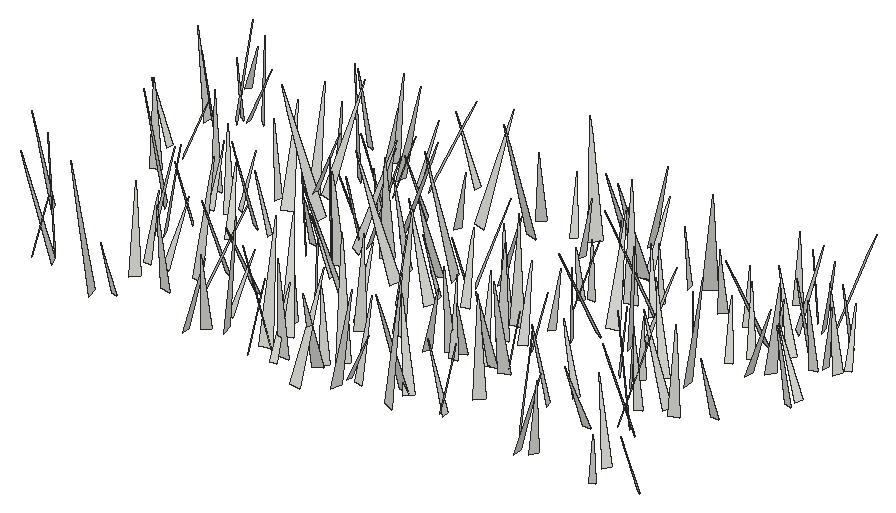
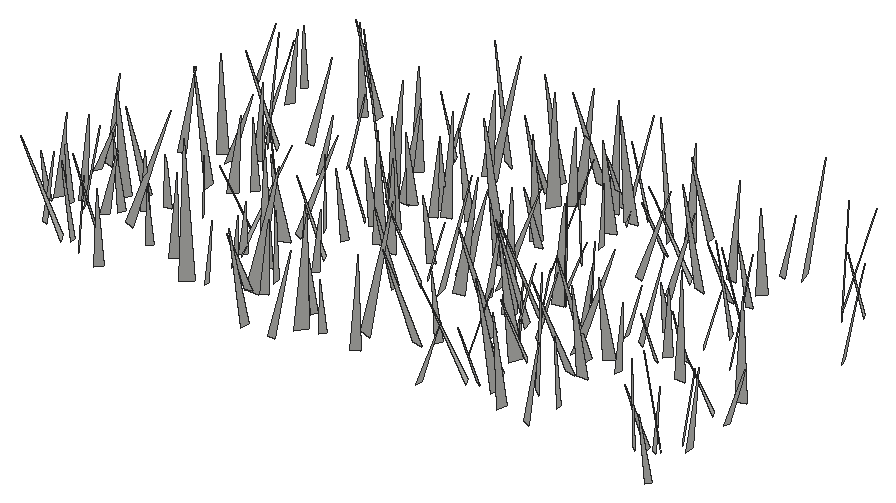
# SketchUp Ruby script. Lengths in inches.
U = 1.inch
M = Sketchup.active_model
def pt(a) = Geom::Point3d.new(a.map { |v| v * U })
def face(e, loops, mat)
  f = e.add_face(loops[0].map { |a| pt(a) })
  loops[1..].each { |l| e.add_face(l.map { |a| pt(a) }).erase! }
  f.material = f.back_material = mat if mat
  f
end
# faces: each face lists its corners as indices into pts; further lists are holes
def faces(e, pts, list, mat = nil) = list.each { |f| face(e, (f[0].is_a?(Array) ? f : [f]).map { |l| l.map { |i| pts[i] } }, mat) }
# xy, xz, yz: faces in a plane at the given z, y or x. An outline is a flat list of corners, or four numbers for a rectangle; further outlines are holes
def ring(l) = l.size == 4 ? [[l[0], l[1]], [l[2], l[1]], [l[2], l[3]], [l[0], l[3]]] : l.each_slice(2).to_a
def flat(e, list, mat, &to3) = list.each { |f| face(e, (f[0].is_a?(Array) ? f : [f]).map { |l| ring(l).map { |u, v| to3.(u, v) } }, mat) }
def xy(e, z, list, mat = nil) = flat(e, list, mat) { |x, y| [x, y, z] }
def xz(e, y, list, mat = nil) = flat(e, list, mat) { |x, z| [x, y, z] }
def yz(e, x, list, mat = nil) = flat(e, list, mat) { |y, z| [x, y, z] }
def lines(e, pts, list) = list.each { |a, b| e.add_line(pt(pts[a]), pt(pts[b])) }
# prism: a flat outline (further loops are holes) pulled along v
def prism(e, loops, v, mat = nil)
  f = face(e, loops, mat); d = Geom::Vector3d.new(v.map { |x| x * U })
  f.pushpull(f.normal.samedirection?(d) ? d.length : -d.length)
end
def box(e, o, s, mat = nil) = prism(e, [[o, [o[0] + s[0], o[1], o[2]], [o[0] + s[0], o[1] + s[1], o[2]], [o[0], o[1] + s[1], o[2]]]], [0, 0, s[2]], mat)
def at(x, y, z, deg = 0) = Geom::Transformation.translation(pt([x, y, z])) * Geom::Transformation.rotation(ORIGIN, Z_AXIS, deg.degrees)
def axes(o, x, y, z) = Geom::Transformation.new([*x, 0, *y, 0, *z, 0, *pt(o).to_a, 1])
def part(name) = M.definitions.add(name)
# library, detail: a bought-in or finely detailed component or shape, given as its bounding box
def library(name, o, s) = part(name).tap { |d| box(d.entities, o, s) }
def detail(e, o, s) = box(e.add_group.entities, o, s)
def put(e, d, t, mat = nil) = e.add_instance(d, t).tap { |i| i.material = mat if mat }
def group(e, t, mat = nil) = e.add_group.tap { |g| g.transformation = t; g.material = mat if mat }.entities
root = M.entities
c1 = part("fur_instance\#9")
p = [[0.8125,0,1.79],[0.67,-0.02,1.48],[0,-0.11,0],[0,0.11,0]]
faces(c1.entities,p,[[0,1,2,3]])
put(root,c1,axes([471.78,258.29,-21.66],[-7.67624,-2.38765,2.18106],[-2.53698,7.93,-0.24775],[2.0054,0.89261,8.03519]))
put(root,c1,axes([502.64,255.98,-21.66],[0.72086,7.11073,0.81641],[7.15729,-0.71063,-0.13028],[0.04812,-0.82534,7.14599]))
put(root,c1,axes([485.32,258.2,-21.66],[5.08569,0.11573,0.95874],[0.07501,-5.17107,0.22632],[-0.96278,0.20845,5.08197]))
put(root,c1,axes([502,260.93,-21.66],[2.77965,-6.05851,0.20454],[-6.05263,-2.78627,-0.276],[-0.3362,0.0706,6.66001]))
put(root,c1,axes([486.8125,259.98,-21.66],[3.24454,-4.71501,1.03025],[-4.7617,-3.32972,-0.24278],[-0.78672,0.70811,5.71834]))
put(root,c1,axes([506.35,258.77,-21.66],[6.38697,-1.69717,1.73981],[-1.81592,-6.58358,0.24416],[-1.61547,0.69051,6.6041]))
put(root,c1,axes([473.87,259.71,-21.66],[-0.63245,-3.70623,0.66325],[-3.76509,0.62047,-0.12308],[-0.01169,0.67448,3.75779]))
put(root,c1,axes([542.48,259.39,-21.66],[1.6475,-3.20979,0.84583],[-3.31321,-1.64761,0.20101],[-0.20196,0.8456,3.6023]))
put(root,c1,axes([493.76,258.83,-21.66],[4.05853,2.67005,1.15678],[2.78357,-4.14094,-0.20805],[-0.84796,-0.81387,4.85361]))
put(root,c1,axes([497.67,260.2,-21.66],[0.14601,-6.62439,2.10053],[-6.94709,-0.08453,0.21629],[0.18059,2.1039,6.62247]))
put(root,c1,axes([531.47,259.7,-21.66],[5.98361,0.11352,0.76596],[0.13466,-6.02993,-0.15823],[-0.76252,-0.17402,5.9826]))
put(root,c1,axes([513.71,258.82,-21.66],[3.41828,7.22194,2.57308],[7.56489,-3.63472,0.1519],[-1.24484,-2.25703,7.98861]))
put(root,c1,axes([533.1875,260.57,-21.66],[4.53528,-3.04969,1.17101],[-3.07507,-4.66168,-0.23091],[-1.10265,0.45689,5.46041]))
put(root,c1,axes([495.05,261.21,-21.66],[-4.80805,-4.95386,1.3489],[-5.02147,4.92244,0.17909],[1.0701,0.84054,6.90116]))
put(root,c1,axes([497.5,258.59,-21.66],[-0.4926,4.67354,0.05511],[4.67276,0.49124,0.10792],[-0.10156,-0.0661,4.69819]))
put(root,c1,axes([513.0625,262.56,-21.66],[-2.01035,-7.12989,1.00319],[-7.18316,2.0575,0.22838],[0.49393,0.90254,7.40437]))
put(root,c1,axes([547.67,261.16,-21.66],[-2.17535,-3.01047,0.60266],[-3.06621,2.16789,-0.23847],[0.15643,0.62897,3.70651]))
put(root,c1,axes([463.9,261.31,-21.66],[-6.35383,-3.10693,1.06991],[-3.1587,6.41685,-0.12448],[0.9057,0.58302,7.07168]))
put(root,c1,axes([488.82,261.16,-21.66],[7.15031,1.42356,2.57616],[1.59453,-7.56218,-0.24693],[-2.47399,-0.75958,7.28646]))
put(root,c1,axes([506.3,261.12,-21.66],[3.59656,-0.31618,0.04156],[-0.31764,-3.59357,0.14939],[-0.02828,0.15246,3.60734]))
put(root,c1,axes([519.87,261.36,-21.66],[-4.57594,-0.69447,0.70937],[-0.73517,4.61906,-0.2203],[0.6671,0.32667,4.62309]))
put(root,c1,axes([461.07,261.14,-21.66],[3.50621,1.98379,0.78234],[2.0421,-3.55715,-0.13217],[-0.61424,-0.50223,4.02634]))
put(root,c1,axes([502.26,261.875,-21.66],[2.60909,-3.89298,2.22887],[-4.24925,-2.97119,-0.21539],[-1.4377,1.71676,4.68148]))
put(root,c1,axes([507.89,260.87,-21.66],[0.83118,5.18677,1.07004],[5.28228,-0.88982,0.21009],[-0.38088,-1.02179,5.24874]))
put(root,c1,axes([519,261.65,-21.66],[-3.23487,-1.73884,2.61208],[-2.22596,3.91581,-0.14997],[2.2117,1.39779,3.66954]))
put(root,c1,axes([494.65,260.86,-21.66],[-1.18605,7.62635,1.82441],[7.84154,1.15487,0.27022],[0.00582,-1.84431,7.7133]))
put(root,c1,axes([513.9,262.27,-21.66],[-4.47005,3.93119,1.60818],[4.11701,4.5843,0.23722],[1.04438,-1.24571,5.94805]))
put(root,c1,axes([462.84,262.94,-21.66],[-5.77727,-4.35757,2.82703],[-4.73437,6.15702,-0.18467],[2.13687,1.8601,7.23403]))
put(root,c1,axes([477.77,263.97,-21.66],[-0.39451,-5.89979,1.57703],[-6.09619,0.47415,0.24879],[0.36204,1.55494,5.90773]))
put(root,c1,axes([528.8,263.52,-21.66],[5.52113,3.74347,2.2115],[4.00437,-5.77059,-0.2291],[-1.6939,-1.44011,6.66663]))
put(root,c1,axes([541.49,263.27,-21.66],[-4.9618,2.41645,1.1014],[2.44275,5.06865,-0.11597],[1.04177,-0.37582,5.51772]))
put(root,c1,axes([503.73,263.29,-21.66],[5.91163,-3.56463,4.13587],[-4.286,-6.80601,0.26026],[-3.38262,2.39395,6.89828]))
put(root,c1,axes([473.07,264.4375,-21.66],[3.99343,-3.31881,2.86458],[-3.84361,-4.5142,0.12826],[-2.10878,1.94301,5.19091]))
put(root,c1,axes([487.09,264,-21.66],[1.39427,3.92432,0.17719],[3.92808,-1.39069,-0.10895],[0.04345,-0.20342,4.16322]))
put(root,c1,axes([495.04,264.1,-21.66],[-2.95766,6.66869,1.17233],[6.76114,2.97762,0.11972],[0.36439,-1.12067,7.29416]))
put(root,c1,axes([520.61,266.57,-21.66],[4.6761,-4.10232,2.76945],[-4.45315,-5.14998,-0.1096],[-2.16064,1.73593,6.21956]))
put(root,c1,axes([533.99,269.05,-21.66],[0.26999,-5.16111,0.17986],[-5.16087,-0.27616,-0.17741],[-0.18667,0.17024,5.16512]))
put(root,c1,axes([493.77,267.14,-21.66],[-4.03311,-0.04964,1.55556],[-0.10181,4.31995,-0.1261],[1.55302,0.15428,4.03144]))
put(root,c1,axes([486.14,270.02,-21.66],[-1.09873,-5.30096,0.04279],[-5.29764,1.09638,-0.20521],[-0.19227,0.08352,5.40974]))
put(root,c1,axes([481.14,266.94,-21.66],[5.4364,3.24485,0.19999],[3.25087,-5.4295,-0.27539],[-0.03035,-0.33899,6.32516]))
put(root,c1,axes([472.36,267.56,-21.66],[0.52075,4.40411,1.27547],[4.58416,-0.47433,-0.2338],[0.09203,-1.29345,4.42863]))
put(root,c1,axes([474.73,267.89,-21.66],[0.96438,4.41888,0.40988],[4.43511,-0.94495,-0.24768],[0.15571,-0.45288,4.5161]))
put(root,c1,axes([479.1,267.98,-21.66],[1.99412,7.08431,1.8343],[7.27705,-2.12036,0.27805],[-0.77249,-1.68678,7.35436]))
put(root,c1,axes([538.9,271.21,-21.66],[-4.24041,-4.62675,0.86788],[-4.65391,4.29598,0.16351],[0.70788,0.52807,6.27385]))
put(root,c1,axes([480.99,271.25,-21.66],[-2.16973,-4.86696,0.63571],[-4.9077,2.16207,-0.19771],[0.07681,0.6613,5.32503]))
put(root,c1,axes([456.41,270.67,-21.66],[-5.55068,-3.03255,1.58004],[-3.06213,5.7489,0.27653],[1.52193,0.50669,6.31901]))
put(root,c1,axes([500.48,270.44,-21.66],[3.75494,-4.9741,2.2471],[-5.32599,-3.93562,0.18806],[-1.1937,1.91308,6.22943]))
put(root,c1,axes([527.41,270.4,-21.66],[-4.67685,-1.64881,1.07356],[-1.71505,4.77313,-0.14071],[0.96421,0.49258,4.95698]))
put(root,c1,axes([509.15,271.6,-21.66],[4.77577,-2.2799,0.31782],[-2.26651,-4.78515,-0.26858],[-0.40236,-0.10607,5.28524]))
put(root,c1,axes([519.17,272.82,-21.66],[2.40943,-6.40182,1.38295],[-6.51779,-2.4885,-0.16399],[-0.64358,1.23501,6.83826]))
put(root,c1,axes([493.33,271.34,-21.66],[2.79577,3.11606,1.7882],[3.42019,-3.00212,-0.11591],[-1.09992,-1.41467,4.18482]))
put(root,c1,axes([517.26,273.11,-21.66],[0.8568,-5.86099,0.80486],[-5.91149,-0.87995,-0.11477],[-0.231,0.77949,5.92218]))
put(root,c1,axes([511.58,272.625,-21.66],[1.49133,-6.04191,1.54576],[-6.23212,-1.50337,0.13646],[-0.23383,1.53405,6.22175]))
put(root,c1,axes([512.8125,273.37,-21.66],[2.32528,-3.90872,0.2043],[-3.90658,-2.33236,-0.15975],[-0.24182,0.09371,4.54527]))
put(root,c1,axes([537.51,272.17,-21.66],[-5.07554,-4.81191,2.50581],[-5.17107,5.32884,-0.24106],[1.64121,1.90882,6.98981]))
put(root,c1,axes([512.68,271.76,-21.66],[-0.37436,4.96388,1.61425],[5.21969,0.34743,0.14211],[-0.02763,-1.62026,4.97594]))
put(root,c1,axes([536.22,271.91,-21.66],[5.52496,2.9641,0.73245],[3.00682,-5.54515,-0.24054],[-0.53047,-0.55942,6.26523]))
put(root,c1,axes([499.2,271.52,-21.66],[-0.62067,4.74172,0.56344],[4.77083,0.63973,-0.12835],[0.20124,-0.5417,4.78044]))
put(root,c1,axes([504.53,272.24,-21.66],[0.76042,7.54721,2.45249],[7.93568,-0.724,-0.23253],[-0.00259,-2.46349,7.58186]))
put(root,c1,axes([495.14,274.3,-21.66],[-6.81995,-3.62088,0.84533],[-3.65528,6.85252,-0.13797],[0.68141,0.51893,7.72033]))
put(root,c1,axes([468.87,272.86,-21.66],[3.65147,4.43575,1.22236],[4.5601,-3.69672,-0.20725],[-0.61278,-1.07778,5.74161]))
put(root,c1,axes([516.36,272.67,-21.66],[-2.91757,4.706,0.99504],[4.75363,2.9987,-0.24403],[0.73452,-0.71423,5.53165]))
put(root,c1,axes([518.86,273.82,-21.66],[3.30079,2.00098,0.99665],[2.11543,-3.37049,-0.23912],[-0.72261,-0.72685,3.85253]))
put(root,c1,axes([528.85,273.5,-21.66],[-4.50468,1.1443,0.55643],[1.12699,4.53841,-0.20945],[0.5907,0.0676,4.64302]))
put(root,c1,axes([469.8,274,-21.66],[5.42096,2.25752,1.64956],[2.38588,-5.61122,-0.16143],[-1.45775,-0.7887,5.87002]))
put(root,c1,axes([536.05,275.6,-21.66],[-1.45922,4.42701,2.15741],[4.90506,1.50733,0.22462],[0.43952,-2.12407,4.65589]))
put(root,c1,axes([540.0625,276.96,-21.66],[2.8988,-5.16102,2.16058],[-5.5292,-3.01461,0.21733],[-0.85564,1.9958,5.91539]))
put(root,c1,axes([470.66,277.77,-21.66],[-3.26871,-2.2439,0.63682],[-2.29753,3.28654,-0.21245],[0.40248,0.53729,3.95909]))
put(root,c1,axes([490.34,277.99,-21.66],[-3.97846,-0.22397,0.26493],[-0.21326,3.98441,0.16592],[0.27363,-0.15114,3.9813]))
put(root,c1,axes([543.85,279.51,-21.66],[0.47232,-5.02453,0.37853],[-5.03579,-0.45765,0.20889],[0.17316,0.39615,5.04235]))
put(root,c1,axes([514.4,278.42,-21.66],[4.01557,-5.25956,2.05629],[-5.53772,-4.16187,0.169],[-1.10676,1.74125,6.61508]))
put(root,c1,axes([500.37,277.47,-21.66],[0.04059,4.23783,1.33242],[4.44047,0.00019,-0.13586],[0.12965,-1.33303,4.23585]))
put(root,c1,axes([538.44,277.81,-21.66],[-5.80532,1.01557,0.17125],[1.00882,5.80466,-0.22508],[0.20737,0.19232,5.88918]))
put(root,c1,axes([465.71,279.17,-21.66],[-6.16765,-3.82155,1.90605],[-3.98751,6.35208,-0.16723],[1.52874,1.15063,7.2537]))
put(root,c1,axes([532.24,278.93,-21.66],[-2.65775,-2.55388,1.91088],[-2.80676,3.05414,0.17806],[1.51521,1.17784,3.68161]))
put(root,c1,axes([476.0625,277.5625,-21.66],[-2.52047,3.62206,0.22803],[3.61381,2.53037,-0.24846],[0.33426,-0.04477,4.40572]))
put(root,c1,axes([489.03,279.4,-21.66],[4.97701,4.02381,2.97396],[4.34378,-5.5566,0.24873],[-2.48337,-1.65505,6.3953]))
put(root,c1,axes([518.21,278.93,-21.66],[2.97809,2.23148,0.68885],[2.24903,-3.04112,0.12836],[-0.62921,-0.30835,3.71915]))
put(root,c1,axes([489.35,280.5,-21.66],[1.40139,-5.88916,2.09043],[-6.21682,-1.53152,-0.14692],[-0.635,1.99706,6.05182]))
put(root,c1,axes([516.77,279.16,-21.66],[-2.07994,4.49979,1.08625],[4.57933,2.1742,-0.23818],[0.67657,-0.88257,4.95151]))
put(root,c1,axes([484.82,280.3,-21.66],[-3.86454,-2.68359,1.87384],[-2.96857,4.09497,-0.25773],[1.3786,1.29506,4.69786]))
put(root,c1,axes([502.83,279.78,-21.66],[-5.78073,2.46703,0.60773],[2.49572,5.79658,0.20851],[0.47643,-0.43109,6.28168]))
put(root,c1,axes([476.64,281.57,-21.66],[-2.84226,-5.05917,1.08036],[-5.16298,2.85167,-0.22901],[0.32566,1.05526,5.79838]))
put(root,c1,axes([529.49,280.45,-21.66],[3.10895,3.01642,1.49943],[3.22004,-3.26039,-0.11754],[-0.98914,-1.13301,4.33019]))
put(root,c1,axes([531.97,281.25,-21.66],[2.86459,-3.18276,1.27512],[-3.34476,-2.95943,0.1272],[-0.754,1.03614,4.28015]))
put(root,c1,axes([479.02,281.16,-21.66],[-3.86057,-0.50737,0.50019],[-0.53854,3.88252,-0.21837],[0.46646,0.28336,3.88764]))
put(root,c1,axes([496.76,281.26,-21.66],[-8.06825,0.70999,0.37952],[0.71569,8.07597,0.10667],[0.36866,-0.13964,8.09873]))
put(root,c1,axes([484.07,282.51,-21.66],[-0.05824,-3.81958,0.55077],[-3.85535,0.08183,0.15984],[0.16986,0.54776,3.81668]))
put(root,c1,axes([502.81,281.625,-21.66],[-3.79015,-1.11399,0.60809],[-1.15598,3.82064,-0.20588],[0.52388,0.37109,3.9451]))
put(root,c1,axes([513.49,282.1,-21.66],[-2.45983,6.23998,3.07468],[6.83629,2.77173,-0.15592],[1.28687,-2.79677,6.7055]))
put(root,c1,axes([506.4,281.81,-21.66],[-1.7521,4.37342,1.24469],[4.49457,1.86786,-0.23622],[0.6891,-1.06311,4.7054]))
put(root,c1,axes([511.42,282.86,-21.66],[-0.9402,5.50023,2.63792],[6.09336,0.97222,0.14463],[0.28664,-2.62629,5.57814]))
put(root,c1,axes([470.32,281.48,-21.66],[0.12612,4.07155,0.3622],[4.08216,-0.1442,0.19951],[-0.2114,-0.35539,4.06861]))
put(root,c1,axes([499.63,285.38,-21.66],[2.0561,-6.44135,0.2848],[-6.4395,-2.06652,-0.24899],[-0.32395,0.19535,6.75697]))
put(root,c1,axes([472.42,282.07,-21.66],[-4.08375,3.22336,1.0157],[3.24667,4.18417,-0.22495],[0.93853,-0.4488,5.19774]))
put(root,c1,axes([520.35,283.38,-21.66],[4.15283,1.56186,1.94961],[1.7605,-4.5132,-0.13443],[-1.7723,-0.82343,4.43479]))
put(root,c1,axes([536.68,283.61,-21.66],[7.17764,0.6661,2.04171],[0.73913,-7.45363,-0.1667],[-2.01642,-0.36113,7.20655]))
put(root,c1,axes([517.06,283.875,-21.66],[3.70956,-2.15387,1.10856],[-2.28011,-3.78925,0.26761],[-0.81802,0.79458,4.28116]))
put(root,c1,axes([496.37,284.1,-21.66],[-5.73495,-0.11109,1.68244],[-0.04447,5.97258,0.24275],[1.68552,-0.22038,5.73089]))
put(root,c1,axes([533.68,283.11,-21.66],[-4.18107,4.06515,1.12452],[4.17237,4.21812,0.26475],[0.61747,-0.97641,5.82552]))
put(root,c1,axes([521.83,286.21,-21.66],[-3.10911,-5.59083,0.18925],[-5.58666,3.11434,0.22319],[0.28707,0.05678,6.39328]))
put(root,c1,axes([492.43,285.25,-21.66],[4.53182,-5.76132,1.66498],[-5.89155,-4.66684,-0.11276],[-1.12014,1.237,7.32923]))
put(root,c1,axes([504.39,284.9,-21.66],[-3.02688,-2.08558,0.64094],[-2.07151,3.09116,0.27563],[0.68504,0.13224,3.66547]))
put(root,c1,axes([459.58,284.98,-21.66],[2.04038,-5.82637,1.87095],[-6.1057,-2.07021,0.21174],[-0.4092,1.83789,6.16967]))
put(root,c1,axes([472.86,283.49,-21.66],[1.48501,3.27806,0.44782],[3.28348,-1.52047,0.24164],[-0.40618,-0.30651,3.59062]))
put(root,c1,axes([468,285.37,-21.66],[0.12589,-6.48138,2.39431],[-6.90548,-0.03647,0.26437],[0.23531,2.39734,6.47721]))
put(root,c1,axes([501.4,286.3,-21.66],[-7.78363,-1.77881,1.5879],[-1.77027,7.9428,0.22014],[1.59741,0.13482,7.98126]))
put(root,c1,axes([548.46,286.83,-21.66],[-1.20745,-5.31811,1.49773],[-5.50418,1.29079,0.14593],[0.47907,1.42653,5.45151]))
put(root,c1,axes([526.46,286.16,-21.66],[-5.78196,-1.74059,3.08913],[-1.82129,6.52793,0.26926],[3.04225,0.59997,6.03227]))
put(root,c1,axes([487.04,286.9375,-21.66],[2.58883,2.26123,2.35644],[2.87323,-3.00647,-0.27159],[-1.55259,-1.79333,3.42658]))
put(root,c1,axes([488.87,284.19,-21.66],[3.08355,6.47581,0.56476],[6.50039,-3.07095,-0.27862],[0.00972,-0.62967,7.16706]))
put(root,c1,axes([489.17,286.17,-21.66],[6.39922,1.66084,0.77373],[1.68967,-6.43637,-0.15871],[-0.70856,-0.34898,6.60932]))
put(root,c1,axes([486.41,287.93,-21.66],[-2.51428,-3.3921,0.48717],[-3.39486,2.54791,0.21985],[0.4675,0.25907,4.21659]))
put(root,c1,axes([481.19,287.43,-21.66],[-8.2127,0.65784,0.53458],[0.66874,8.22786,0.14871],[0.52088,-0.19122,8.23766]))
put(root,c1,axes([504.21,286.4,-21.66],[4.71146,3.59222,0.48874],[3.58656,-4.73541,0.23065],[-0.52868,-0.11206,5.92019]))
put(root,c1,axes([478.84,288.17,-21.66],[6.32916,0.13104,0.27334],[0.13733,-6.3333,-0.14369],[-0.27023,-0.14945,6.32889]))
put(root,c1,axes([477.09,286.64,-21.66],[-2.49742,5.95651,1.04282],[6.02179,2.55284,-0.16018],[0.55273,-0.89868,6.45689]))
put(root,c1,axes([474.625,288.1,-21.66],[-4.53937,1.16522,1.40638],[1.15678,4.75002,-0.2018],[1.41333,-0.14527,4.6822]))
put(root,c1,axes([516.41,288.28,-21.66],[4.75078,2.28793,0.55209],[2.32197,-4.75936,-0.25743],[-0.38451,-0.47246,5.26671]))
put(root,c1,axes([506.1,288.59,-21.66],[4.91416,0.05831,0.74386],[0.02898,-4.96646,0.19783],[-0.74558,0.19125,4.91052]))
put(root,c1,axes([548.78,288.45,-21.66],[-4.27711,1.68369,0.0136],[1.68167,4.26988,0.26227],[-0.08344,-0.24902,4.58909]))
put(root,c1,axes([533.05,289.13,-21.66],[3.08289,1.97486,1.70839],[2.08981,-3.45082,0.21788],[-1.56569,-0.71742,3.6547]))
put(root,c1,axes([540.625,289.69,-21.66],[5.32067,-0.59583,0.38531],[-0.58759,-5.33383,-0.13414],[-0.39777,-0.09079,5.35224]))
put(root,c1,axes([487.4,289.77,-21.66],[2.96101,1.91002,1.7712],[2.18546,-3.28075,-0.11568],[-1.41742,-1.06838,3.5217]))
put(root,c1,axes([526.92,288.35,-21.66],[2.95968,3.81178,0.17357],[3.80838,-2.96454,0.16477],[-0.23661,-0.0359,4.82309]))
put(root,c1,axes([457.63,289.93,-21.66],[-4.13289,0.76106,0.51137],[0.79822,4.14817,0.27763],[0.45116,-0.36746,4.1932]))
put(root,c1,axes([460.37,288.99,-21.66],[3.48298,2.03603,0.22687],[2.02285,-3.48877,0.25421],[-0.32396,0.10555,4.02641]))
put(root,c1,axes([522.31,288.27,-21.66],[-2.78795,6.31949,0.96814],[6.36227,2.84625,-0.25738],[0.62828,-0.78026,6.90234]))
put(root,c1,axes([515.3,291.33,-21.66],[2.03457,-2.99845,1.01926],[-3.06758,-2.16697,-0.25148],[-0.78708,0.69471,3.61482]))
put(root,c1,axes([490.62,290.35,-21.66],[6.76067,1.19839,0.69108],[1.18973,-6.79585,0.14582],[-0.7059,0.02372,6.86451]))
put(root,c1,axes([542.37,291.33,-21.66],[5.43979,-3.16023,1.66658],[-3.30816,-5.60189,0.17546],[-1.34931,0.9938,6.28869]))
put(root,c1,axes([537.27,290.32,-21.66],[-1.47,3.64091,0.87512],[3.73843,1.4809,0.11844],[0.21496,-0.85654,3.92467]))
put(root,c1,axes([486.72,292.14,-21.66],[-4.48858,-3.56813,1.07524],[-3.58767,4.5928,0.2643],[1.00813,0.45789,5.72792]))
put(root,c1,axes([524.41,293.26,-21.66],[-5.605,-5.08718,0.25266],[-5.09303,5.60246,-0.18084],[0.06544,0.30374,7.56721]))
put(root,c1,axes([516.32,291.875,-21.66],[0.16475,-3.83195,1.51207],[-4.1166,-0.0965,0.20397],[0.15418,1.51796,3.83006]))
put(root,c1,axes([485.19,293.2,-21.66],[6.75458,-3.1446,1.55563],[-3.25939,-6.87331,0.25842],[-1.29802,0.89549,7.44621]))
put(root,c1,axes([476.94,291.55,-21.66],[-0.4945,6.57851,1.5324],[6.75453,0.47319,0.14829],[-0.03697,-1.53911,6.5954]))
put(root,c1,axes([538.65,292.53,-21.66],[-2.21571,3.96483,0.99922],[4.07213,2.24229,0.13245],[0.36886,-0.93805,4.54001]))
put(root,c1,axes([538.22,296.03,-21.66],[-2.55623,-6.61752,0.06611],[-6.61278,2.55692,0.25211],[0.25899,-0.02922,7.08959]))
put(root,c1,axes([484.28,292.34,-21.66],[3.52648,2.43175,0.31475],[2.41999,-3.54045,0.23962],[-0.3951,0.0194,4.27692]))
put(root,c1,axes([540.69,294.29,-21.66],[4.29298,-1.68508,0.76366],[-1.68331,-4.35833,-0.1541],[-0.76754,0.13347,4.60928]))
put(root,c1,axes([545.64,294.87,-21.66],[1.04102,-4.92803,1.21287],[-5.07408,-1.03535,0.14838],[-0.10125,1.21771,5.0346]))
put(root,c1,axes([524.11,293.21,-21.66],[-2.51117,3.39602,0.58609],[3.43959,2.51478,0.1658],[0.21361,-0.57041,4.22035]))
put(root,c1,axes([478.67,291.68,-21.66],[1.55056,7.17303,0.47228],[7.18686,-1.53634,-0.26142],[0.15632,-0.51668,7.33405]))
put(root,c1,axes([490.3125,295.12,-21.66],[-3.61255,-2.36918,0.54232],[-2.35627,3.65218,0.25916],[0.59592,0.07847,4.31235]))
put(root,c1,axes([520.34,293.97,-21.66],[1.64686,-6.77743,3.62945],[-7.62252,-1.92308,-0.13234],[-1.0018,3.49096,6.97339]))
put(root,c1,axes([494.48,295.4,-21.66],[4.0424,-1.6774,0.68877],[-1.67315,-4.09915,-0.16314],[-0.69903,0.11126,4.37357]))
put(root,c1,axes([544.71,295.8,-21.66],[-4.89111,-2.11302,1.38613],[-2.21595,5.03778,-0.13961],[1.21481,0.68196,5.3262]))
put(root,c1,axes([517.23,295.9,-21.66],[4.14484,0.5886,1.74948],[0.68446,-4.48393,-0.11303],[-1.71425,-0.36717,4.1849]))
put(root,c1,axes([546.34,296.25,-21.66],[4.13906,-0.88394,1.08396],[-0.87234,-4.27812,-0.15771],[-1.09332,0.06702,4.22946]))
put(root,c1,axes([548.3,295.96,-21.66],[-4.8782,2.33838,1.88669],[2.5546,5.12175,0.25721],[1.58166,-1.06025,5.40358]))
put(root,c1,axes([458.8125,296.27,-21.66],[3.31439,2.62679,2.62231],[3.03004,-3.94532,0.12232],[-2.14367,-1.5153,4.22732]))
put(root,c1,axes([523.06,296.1,-21.66],[3.01506,-0.72225,2.0256],[-1.00024,-3.559,0.21985],[-1.90373,0.72607,3.09256]))
put(root,c1,axes([541.875,295.73,-21.66],[-4.34264,3.05124,0.46122],[3.07623,4.34339,0.23041],[0.24406,-0.45414,5.3024]))
put(root,c1,axes([478.83,297.26,-21.66],[-4.49865,-5.44108,2.87885],[-5.83326,4.90701,0.15896],[1.96626,2.10876,7.05818]))
put(root,c1,axes([502.04,299.03,-21.66],[-2.39726,-7.68863,1.50052],[-7.81274,2.46126,0.12966],[0.5725,1.39306,8.05265]))
put(root,c1,axes([517.87,299.44,-21.66],[0.49777,-7.47829,0.86543],[-7.52286,-0.52678,-0.22508],[-0.28353,0.84808,7.49146]))
put(root,c1,axes([457.3,297.07,-21.66],[4.90342,0.51596,3.18153],[0.4361,-5.84514,0.27581],[-3.19346,-0.00597,4.92277]))
put(root,c1,axes([484.25,296.61,-21.66],[3.13129,2.44329,0.37399],[2.42945,-3.15346,0.26073],[-0.45532,-0.0231,3.96316]))
put(root,c1,axes([529.62,298.79,-21.66],[3.06125,-3.87557,0.82155],[-3.90702,-3.12527,-0.1848],[-0.65588,0.52812,4.93529]))
put(root,c1,axes([474.8,298.45,-21.66],[4.07501,0.67414,1.38281],[0.80205,-4.27202,-0.28088],[-1.31276,-0.5174,4.12083]))
put(root,c1,axes([548.76,297.29,-21.66],[-1.59242,3.59476,0.56652],[3.61736,1.63113,-0.18207],[0.39739,-0.44291,3.92746]))
put(root,c1,axes([533.58,298.15,-21.66],[-2.47,2.58512,1.49197],[2.74392,2.72878,-0.18549],[1.17462,-0.93843,3.57063]))
put(root,c1,axes([509.375,299,-21.66],[4.26328,-1.39926,0.74192],[-1.39292,-4.32659,-0.15583],[-0.75375,0.08115,4.48433]))
put(root,c1,axes([516.62,298.9,-21.66],[2.27684,-3.73592,1.683],[-3.94498,-2.51908,-0.25488],[-1.10756,1.29258,4.36763]))
put(root,c1,axes([496.08,297.24,-21.66],[1.83288,7.01444,0.75411],[7.05484,-1.82448,-0.17632],[-0.01908,-0.77421,7.24781]))
put(root,c1,axes([460.07,299.89,-21.66],[-1.89592,-3.45095,1.30694],[-3.60556,2.04518,0.16982],[0.78554,1.05823,3.9338]))
put(root,c1,axes([459.89,298.97,-21.66],[-4.21577,-3.58718,3.5566],[-4.31781,4.96325,-0.11214],[2.62178,2.40587,5.53425]))
put(root,c1,axes([482.59,300.03,-21.66],[6.6153,-1.38256,1.33275],[-1.44359,-6.733,0.18083],[-1.26639,0.45296,6.75581]))
put(root,c1,axes([525.23,301.94,-21.66],[5.72891,-5.77899,0.7373],[-5.79412,-5.75966,-0.12335],[-0.60698,0.43635,8.13646]))
put(root,c1,axes([460.98,299.86,-21.66],[4.07736,0.20577,0.16386],[0.20057,-4.0788,0.13116],[-0.17019,0.12285,4.08044]))
put(root,c1,axes([462.42,300.61,-21.66],[-3.23296,-4.09809,2.47034],[-4.47809,3.64184,0.18098],[1.68632,1.81429,5.21667]))
put(root,c1,axes([523.06,301.07,-21.66],[3.59976,0.06174,1.80471],[0.19659,-4.01441,-0.2548],[-1.79504,-0.31584,3.59126]))
put(root,c1,axes([545.87,301.42,-21.66],[-1.67476,-3.89018,1.26522],[-4.03938,1.78862,0.15259],[0.64624,1.09838,4.23261]))
put(root,c1,axes([485.2,299.96,-21.66],[2.13777,3.57515,0.4757],[3.58502,-2.16686,0.17428],[-0.39447,-0.3179,4.1619]))
put(root,c1,axes([500.69,302.58,-21.66],[3.52243,-4.25283,0.7835],[-4.27225,-3.57882,-0.21878],[-0.66956,0.46198,5.5178]))
put(root,c1,axes([518.39,299.35,-21.66],[-0.5351,4.97369,0.08314],[4.96853,0.53845,-0.2337],[0.24128,-0.05757,4.99693]))
put(root,c1,axes([486.43,300.36,-21.66],[5.74165,3.30721,0.02247],[3.30582,-5.73764,-0.2359],[0.09829,-0.21562,6.62182]))
put(root,c1,axes([538.85,300.56,-21.66],[-2.72966,-3.54913,3.67888],[-4.47058,3.67982,0.23296],[2.47878,2.72838,4.47136]))
put(root,c1,axes([505.9,301.85,-21.66],[-2.49672,2.92464,0.96124],[2.97957,2.60694,-0.1927],[0.77439,-0.6012,3.84057]))
put(root,c1,axes([540.94,302.72,-21.66],[4.61454,1.12705,1.27743],[1.23829,-4.75228,-0.2803],[-1.16993,-0.58453,4.7419]))
put(root,c1,axes([479.63,302.59,-21.66],[5.47744,-1.647,1.93505],[-1.81976,-5.75174,0.25556],[-1.77356,0.81501,5.71398]))
put(root,c1,axes([508.29,302.625,-21.66],[5.58768,-4.04107,3.86555],[-4.58295,-6.44048,-0.10822],[-3.20457,2.16447,6.89498]))
put(root,c1,axes([475.3,303.64,-21.66],[-2.10468,-4.52268,1.53831],[-4.75533,2.14388,-0.20306],[0.45584,1.48319,4.98428]))
put(root,c1,axes([539,304.06,-21.66],[-3.54566,-2.66431,1.6705],[-2.78653,3.82874,0.19209],[1.45754,0.83849,4.43096]))
put(root,c1,axes([490.47,303.95,-21.66],[-4.67838,0.58429,0.4377],[0.60816,4.68963,0.24018],[0.40387,-0.29353,4.7086]))
put(root,c1,axes([509.77,306.17,-21.66],[-0.22883,-5.12281,0.23524],[-5.12454,0.23734,0.18366],[0.19416,0.22665,5.12463]))
put(root,c1,axes([542.21,303.02,-21.66],[6.025,3.41302,0.55167],[3.40656,-6.04972,0.22351],[-0.59027,-0.07668,6.92094]))
put(root,c1,axes([456.22,305.71,-21.66],[3.1539,-2.32332,0.00557],[-2.32207,-3.15188,0.13648],[0.07647,0.11319,3.91488]))
put(root,c1,axes([534.94,305.48,-21.66],[-2.61332,3.50076,2.27341],[3.90248,3.00092,-0.13507],[1.48133,-1.72983,4.36652]))
put(root,c1,axes([513.8,305.88,-21.66],[5.74343,-0.59024,1.12729],[-0.57342,-5.85294,-0.14303],[-1.13593,-0.02976,5.77191]))
